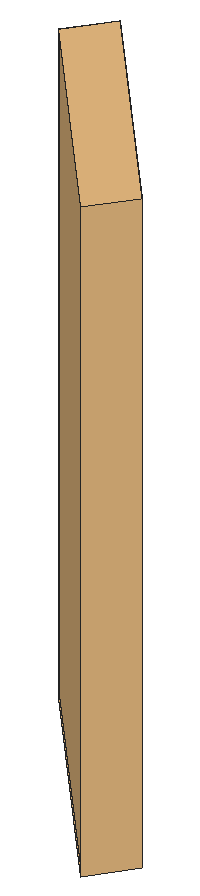
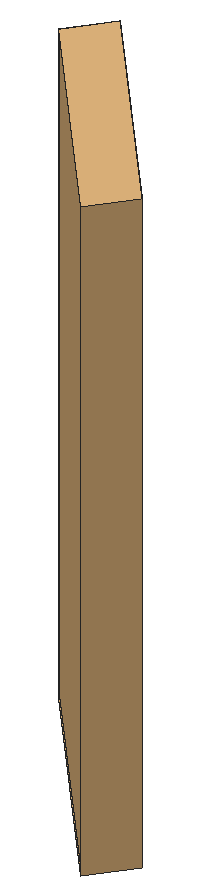
# SketchUp Ruby script. Lengths in inches.
U = 1.inch
M = Sketchup.active_model
def pt(a) = Geom::Point3d.new(a.map { |v| v * U })
def face(e, loops, mat)
  f = e.add_face(loops[0].map { |a| pt(a) })
  loops[1..].each { |l| e.add_face(l.map { |a| pt(a) }).erase! }
  f.material = f.back_material = mat if mat
  f
end
# faces: each face lists its corners as indices into pts; further lists are holes
def faces(e, pts, list, mat = nil) = list.each { |f| face(e, (f[0].is_a?(Array) ? f : [f]).map { |l| l.map { |i| pts[i] } }, mat) }
# xy, xz, yz: faces in a plane at the given z, y or x. An outline is a flat list of corners, or four numbers for a rectangle; further outlines are holes
def ring(l) = l.size == 4 ? [[l[0], l[1]], [l[2], l[1]], [l[2], l[3]], [l[0], l[3]]] : l.each_slice(2).to_a
def flat(e, list, mat, &to3) = list.each { |f| face(e, (f[0].is_a?(Array) ? f : [f]).map { |l| ring(l).map { |u, v| to3.(u, v) } }, mat) }
def xy(e, z, list, mat = nil) = flat(e, list, mat) { |x, y| [x, y, z] }
def xz(e, y, list, mat = nil) = flat(e, list, mat) { |x, z| [x, y, z] }
def yz(e, x, list, mat = nil) = flat(e, list, mat) { |y, z| [x, y, z] }
def lines(e, pts, list) = list.each { |a, b| e.add_line(pt(pts[a]), pt(pts[b])) }
# prism: a flat outline (further loops are holes) pulled along v
def prism(e, loops, v, mat = nil)
  f = face(e, loops, mat); d = Geom::Vector3d.new(v.map { |x| x * U })
  f.pushpull(f.normal.samedirection?(d) ? d.length : -d.length)
end
def box(e, o, s, mat = nil) = prism(e, [[o, [o[0] + s[0], o[1], o[2]], [o[0] + s[0], o[1] + s[1], o[2]], [o[0], o[1] + s[1], o[2]]]], [0, 0, s[2]], mat)
def at(x, y, z, deg = 0) = Geom::Transformation.translation(pt([x, y, z])) * Geom::Transformation.rotation(ORIGIN, Z_AXIS, deg.degrees)
def axes(o, x, y, z) = Geom::Transformation.new([*x, 0, *y, 0, *z, 0, *pt(o).to_a, 1])
def part(name) = M.definitions.add(name)
# library, detail: a bought-in or finely detailed component or shape, given as its bounding box
def library(name, o, s) = part(name).tap { |d| box(d.entities, o, s) }
def detail(e, o, s) = box(e.add_group.entities, o, s)
def put(e, d, t, mat = nil) = e.add_instance(d, t).tap { |i| i.material = mat if mat }
def group(e, t, mat = nil) = e.add_group.tap { |g| g.transformation = t; g.material = mat if mat }.entities
root = M.entities
c1 = library("sm2 st v2 Component\#1",[0,0,0],[29.46,4.93,43.46])
put(root,c1,axes([63.14,104.95,57.27],[0.30765,-0.34028,0],[0.27411,0.38193,0],[0,0,0.6557]))
